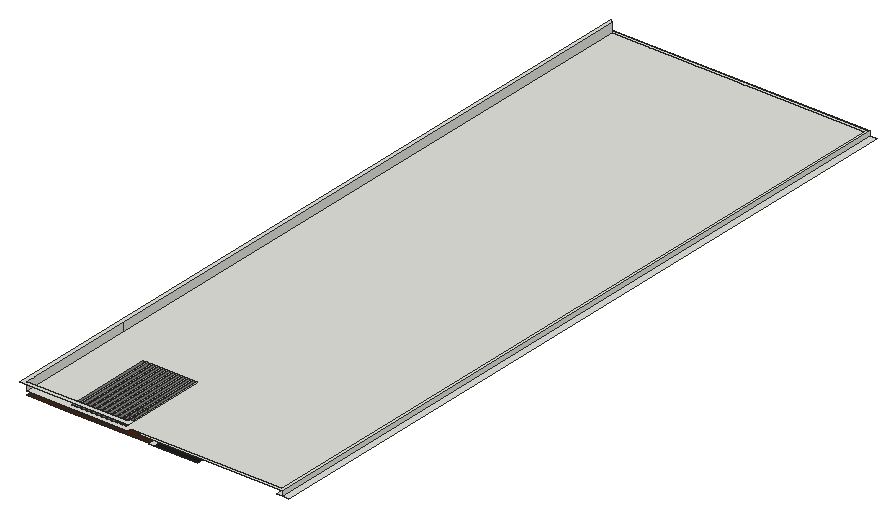
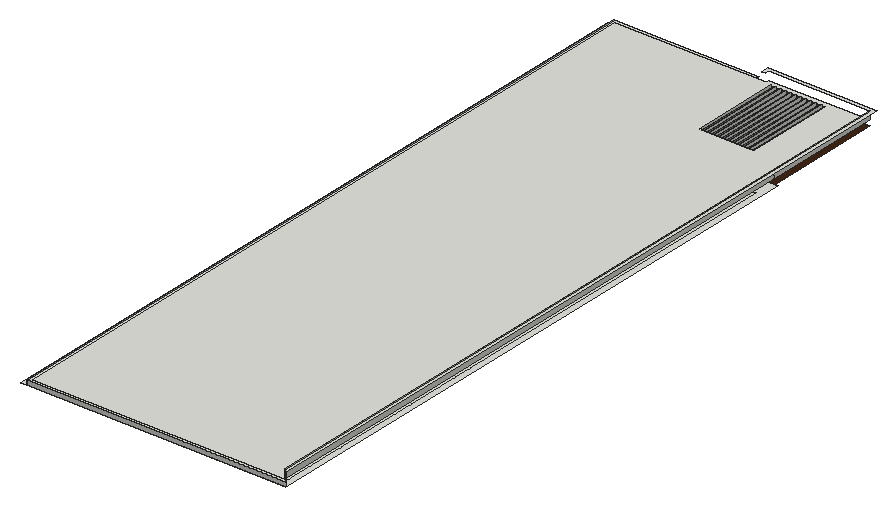
# SketchUp Ruby script. Lengths in inches.
U = 1.inch
M = Sketchup.active_model
def pt(a) = Geom::Point3d.new(a.map { |v| v * U })
def face(e, loops, mat)
  f = e.add_face(loops[0].map { |a| pt(a) })
  loops[1..].each { |l| e.add_face(l.map { |a| pt(a) }).erase! }
  f.material = f.back_material = mat if mat
  f
end
# faces: each face lists its corners as indices into pts; further lists are holes
def faces(e, pts, list, mat = nil) = list.each { |f| face(e, (f[0].is_a?(Array) ? f : [f]).map { |l| l.map { |i| pts[i] } }, mat) }
# xy, xz, yz: faces in a plane at the given z, y or x. An outline is a flat list of corners, or four numbers for a rectangle; further outlines are holes
def ring(l) = l.size == 4 ? [[l[0], l[1]], [l[2], l[1]], [l[2], l[3]], [l[0], l[3]]] : l.each_slice(2).to_a
def flat(e, list, mat, &to3) = list.each { |f| face(e, (f[0].is_a?(Array) ? f : [f]).map { |l| ring(l).map { |u, v| to3.(u, v) } }, mat) }
def xy(e, z, list, mat = nil) = flat(e, list, mat) { |x, y| [x, y, z] }
def xz(e, y, list, mat = nil) = flat(e, list, mat) { |x, z| [x, y, z] }
def yz(e, x, list, mat = nil) = flat(e, list, mat) { |y, z| [x, y, z] }
def lines(e, pts, list) = list.each { |a, b| e.add_line(pt(pts[a]), pt(pts[b])) }
# prism: a flat outline (further loops are holes) pulled along v
def prism(e, loops, v, mat = nil)
  f = face(e, loops, mat); d = Geom::Vector3d.new(v.map { |x| x * U })
  f.pushpull(f.normal.samedirection?(d) ? d.length : -d.length)
end
def box(e, o, s, mat = nil) = prism(e, [[o, [o[0] + s[0], o[1], o[2]], [o[0] + s[0], o[1] + s[1], o[2]], [o[0], o[1] + s[1], o[2]]]], [0, 0, s[2]], mat)
def at(x, y, z, deg = 0) = Geom::Transformation.translation(pt([x, y, z])) * Geom::Transformation.rotation(ORIGIN, Z_AXIS, deg.degrees)
def axes(o, x, y, z) = Geom::Transformation.new([*x, 0, *y, 0, *z, 0, *pt(o).to_a, 1])
def part(name) = M.definitions.add(name)
# library, detail: a bought-in or finely detailed component or shape, given as its bounding box
def library(name, o, s) = part(name).tap { |d| box(d.entities, o, s) }
def detail(e, o, s) = box(e.add_group.entities, o, s)
def put(e, d, t, mat = nil) = e.add_instance(d, t).tap { |i| i.material = mat if mat }
def group(e, t, mat = nil) = e.add_group.tap { |g| g.transformation = t; g.material = mat if mat }.entities
root = M.entities
M.materials.add("[Color M08]").color = [30, 30, 30]
M.materials.add("[Field Square Tile]").color = [211, 167, 108]
M.materials.add("[Granite Light Gray]").color = [149, 148, 144]
M.materials.add("[Wood Veneer 01]").color = [66, 38, 20]
xy(root,380.5,[[1555.29,2346.71,1555.29,3661.44,1107.53,3661.44,1107.53,2597.8,1323.53,2597.8,1323.53,2562.82,1097.72,2562.82,1097.72,3671.25,1565.1,3671.25,1565.1,2346.71],[1323.53,2346.71,1332.45,2425.46],[1565.1,2346.71,1576.91,3671.25],[1323.53,2425.46,1323.53,2597.8,1107.53,2597.8,1107.53,3661.44,1555.29,3661.44,1555.29,2425.46,1508.52,2425.46,1508.52,2532.83,1413.21,2532.83,1413.21,2573.65,1332.45,2573.65,1332.45,2532.83,1323.83,2532.83,1323.83,2425.46],[1323.83,2425.46,1332.45,2532.83],
  [1413.21,2425.46,1508.52,2532.83],[1332.45,2532.83,1413.21,2573.65]])
xy(root,380.5,[[1332.45,2346.71,1413.21,2532.83]],"[Color M08]")
xy(root,380.5,[[[1102.55,2347.9,1174.48,2562.82],[1119.58,2501.63,1121.1,2502.01,1122.48,2502.76,1123.61,2503.84,1124.42,2505.18,1124.85,2506.6875,1124.89,2508.25,1124.51,2509.78,1123.76,2511.15,1122.67,2512.28,1121.33,2513.09,1119.83,2513.53,1118.26,2513.56,1116.74,2513.19,1115.37,2512.43,1114.24,2511.35,1113.43,2510.01,1112.99,2508.5,1112.96,2506.9375,1113.33,2505.41,1114.09,2504.04,1115.17,2502.91,1116.51,2502.1,1118.02,2501.66],[1119.58,2441.63,1121.1,2442.01,1122.48,2442.76,1123.61,2443.84,1124.42,2445.18,1124.85,2446.6875,1124.89,2448.25,1124.51,2449.78,1123.76,2451.15,1122.67,2452.28,1121.33,2453.09,1119.83,2453.53,1118.26,2453.56,1116.74,2453.19,1115.37,2452.43,1114.24,2451.35,1113.43,2450.01,1112.99,2448.5,1112.96,2446.9375,1113.33,2445.41,1114.09,2444.04,1115.17,2442.91,1116.51,2442.1,1118.02,2441.66],[1119.58,2389.88,1121.1,2390.26,1122.48,2391.01,1123.61,2392.09,1124.42,2393.43,1124.85,2394.9375,1124.89,2396.5,1124.51,2398.03,1123.76,2399.4,1122.67,2400.53,1121.33,2401.34,1119.83,2401.78,1118.26,2401.81,1116.74,2401.44,1115.37,2400.68,1114.24,2399.6,1113.43,2398.26,1112.99,2396.75,1112.96,2395.1875,1113.33,2393.66,1114.09,2392.29,1115.17,2391.16,1116.51,2390.35,1118.02,2389.91],[1119.58,2359.13,1121.1,2359.51,1122.48,2360.26,1123.61,2361.34,1124.42,2362.68,1124.85,2364.1875,1124.89,2365.75,1124.51,2367.28,1123.76,2368.65,1122.67,2369.78,1121.33,2370.59,1119.83,2371.03,1118.26,2371.06,1116.74,2370.69,1115.37,2369.93,1114.24,2368.85,1113.43,2367.51,1112.99,2366,1112.96,2364.4375,1113.33,2362.91,1114.09,2361.54,1115.17,2360.41,1116.51,2359.6,1118.02,2359.16],[1159.33,2441.63,1160.85,2442.01,1162.23,2442.76,1163.36,2443.84,1164.17,2445.18,1164.6,2446.6875,1164.64,2448.25,1164.26,2449.78,1163.51,2451.15,1162.42,2452.28,1161.08,2453.09,1159.58,2453.53,1158.01,2453.56,1156.49,2453.19,1155.12,2452.43,1153.99,2451.35,1153.18,2450.01,1152.74,2448.5,1152.71,2446.9375,1153.08,2445.41,1153.84,2444.04,1154.92,2442.91,1156.26,2442.1,1157.77,2441.66],[1159.33,2389.88,1160.85,2390.26,1162.23,2391.01,1163.36,2392.09,1164.17,2393.43,1164.6,2394.9375,1164.64,2396.5,1164.26,2398.03,1163.51,2399.4,1162.42,2400.53,1161.08,2401.34,1159.58,2401.78,1158.01,2401.81,1156.49,2401.44,1155.12,2400.68,1153.99,2399.6,1153.18,2398.26,1152.74,2396.75,1152.71,2395.1875,1153.08,2393.66,1153.84,2392.29,1154.92,2391.16,1156.26,2390.35,1157.77,2389.91],[1159.33,2359.13,1160.85,2359.51,1162.23,2360.26,1163.36,2361.34,1164.17,2362.68,1164.6,2364.1875,1164.64,2365.75,1164.26,2367.28,1163.51,2368.65,1162.42,2369.78,1161.08,2370.59,1159.58,2371.03,1158.01,2371.06,1156.49,2370.69,1155.12,2369.93,1153.99,2368.85,1153.18,2367.51,1152.74,2366,1152.71,2364.4375,1153.08,2362.91,1153.84,2361.54,1154.92,2360.41,1156.26,2359.6,1157.77,2359.16],[1159.33,2501.63,1160.85,2502.01,1162.23,2502.76,1163.36,2503.84,1164.17,2505.18,1164.6,2506.6875,1164.64,2508.25,1164.26,2509.78,1163.51,2511.15,1162.42,2512.28,1161.08,2513.09,1159.58,2513.53,1158.01,2513.56,1156.49,2513.19,1155.12,2512.43,1153.99,2511.35,1153.18,2510.01,1152.74,2508.5,1152.71,2506.9375,1153.08,2505.41,1153.84,2504.04,1154.92,2502.91,1156.26,2502.1,1157.77,2501.66]],[[1174.48,2347.9,1323.53,2562.82],[1269.93,2355.06,1276.18,2516.12],[1260.81,2355.06,1267.06,2516.12],[1251.68,2355.06,1257.93,2516.12],[1242.56,2355.06,1248.81,2516.12],[1233.43,2355.06,1239.68,2516.12],[1224.31,2355.06,1230.56,2516.12],[1215.18,2355.06,1221.43,2516.12],[1206.06,2355.06,1212.31,2516.12],[1196.93,2355.06,1203.18,2516.12],[1187.81,2355.06,1194.06,2516.12],[1178.68,2355.06,1184.93,2516.12]]],"[Wood Veneer 01]")
xy(root,381.875,[[1119.58,2389.88,1118.02,2389.91,1116.51,2390.35,1115.17,2391.16,1114.09,2392.29,1113.33,2393.66,1112.96,2395.1875,1112.99,2396.75,1113.43,2398.26,1114.24,2399.6,1115.37,2400.68,1116.74,2401.44,1118.26,2401.81,1119.83,2401.78,1121.33,2401.34,1122.67,2400.53,1123.76,2399.4,1124.51,2398.03,1124.89,2396.5,1124.85,2394.9375,1124.42,2393.43,1123.61,2392.09,1122.48,2391.01,1121.1,2390.26],[1159.33,2389.88,1157.77,2389.91,1156.26,2390.35,1154.92,2391.16,1153.84,2392.29,1153.08,2393.66,1152.71,2395.1875,1152.74,2396.75,1153.18,2398.26,1153.99,2399.6,1155.12,2400.68,1156.49,2401.44,1158.01,2401.81,1159.58,2401.78,1161.08,2401.34,1162.42,2400.53,1163.51,2399.4,1164.26,2398.03,1164.64,2396.5,1164.6,2394.9375,1164.17,2393.43,1163.36,2392.09,1162.23,2391.01,1160.85,2390.26],[1119.58,2441.63,1118.02,2441.66,1116.51,2442.1,1115.17,2442.91,1114.09,2444.04,1113.33,2445.41,1112.96,2446.9375,1112.99,2448.5,1113.43,2450.01,1114.24,2451.35,1115.37,2452.43,1116.74,2453.19,1118.26,2453.56,1119.83,2453.53,1121.33,2453.09,1122.67,2452.28,1123.76,2451.15,1124.51,2449.78,1124.89,2448.25,1124.85,2446.6875,1124.42,2445.18,1123.61,2443.84,1122.48,2442.76,1121.1,2442.01],[1159.33,2441.63,1157.77,2441.66,1156.26,2442.1,1154.92,2442.91,1153.84,2444.04,1153.08,2445.41,1152.71,2446.9375,1152.74,2448.5,1153.18,2450.01,1153.99,2451.35,1155.12,2452.43,1156.49,2453.19,1158.01,2453.56,1159.58,2453.53,1161.08,2453.09,1162.42,2452.28,1163.51,2451.15,1164.26,2449.78,1164.64,2448.25,1164.6,2446.6875,1164.17,2445.18,1163.36,2443.84,1162.23,2442.76,1160.85,2442.01],[1119.58,2501.63,1118.02,2501.66,1116.51,2502.1,1115.17,2502.91,1114.09,2504.04,1113.33,2505.41,1112.96,2506.9375,1112.99,2508.5,1113.43,2510.01,1114.24,2511.35,1115.37,2512.43,1116.74,2513.19,1118.26,2513.56,1119.83,2513.53,1121.33,2513.09,1122.67,2512.28,1123.76,2511.15,1124.51,2509.78,1124.89,2508.25,1124.85,2506.6875,1124.42,2505.18,1123.61,2503.84,1122.48,2502.76,1121.1,2502.01],
  [1159.33,2501.63,1157.77,2501.66,1156.26,2502.1,1154.92,2502.91,1153.84,2504.04,1153.08,2505.41,1152.71,2506.9375,1152.74,2508.5,1153.18,2510.01,1153.99,2511.35,1155.12,2512.43,1156.49,2513.19,1158.01,2513.56,1159.58,2513.53,1161.08,2513.09,1162.42,2512.28,1163.51,2511.15,1164.26,2509.78,1164.64,2508.25,1164.6,2506.6875,1164.17,2505.18,1163.36,2503.84,1162.23,2502.76,1160.85,2502.01]],"[Field Square Tile]")
xy(root,388.625,[[[1104.06,2346.49,1287.38,2346.49,1287.38,2353.05,1558.75,2353.05,1558.75,3664.91,1104.06,3664.91],[1178.68,2355.06,1184.93,2516.12],[1187.81,2355.06,1194.06,2516.12],[1196.93,2355.06,1203.18,2516.12],[1206.06,2355.06,1212.31,2516.12],[1215.18,2355.06,1221.43,2516.12],[1224.31,2355.06,1230.56,2516.12],[1233.43,2355.06,1239.68,2516.12],[1242.56,2355.06,1248.81,2516.12],[1251.68,2355.06,1257.93,2516.12],[1260.81,2355.06,1267.06,2516.12],[1269.93,2355.06,1276.18,2516.12]],[1304.4375,2346.71,1565.1,2346.71,1565.1,3671.25,1097.72,3671.25,1104.06,3664.91,1558.75,3664.91,1558.75,2353.05,1304.4375,2353.05]])
xy(root,403.8125,[[1097.72,2340.15,1293.73,2340.15,1293.73,2353.05,1287.38,2353.05,1287.38,2346.49,1104.06,2346.49,1104.06,3664.91,1097.72,3671.25]])
xz(root,2516.12,[[1178.68,380.5,1184.93,388.625],[1187.81,380.5,1194.06,388.625],[1196.93,380.5,1203.18,388.625],[1206.06,380.5,1212.31,388.625],[1215.18,380.5,1221.43,388.625],
  [1224.31,380.5,1230.56,388.625],[1233.43,380.5,1239.68,388.625],[1242.56,380.5,1248.81,388.625],[1251.68,380.5,1257.93,388.625],[1260.81,380.5,1267.06,388.625],
  [1269.93,380.5,1276.18,388.625]],"[Granite Light Gray]")
xz(root,3671.25,[[1097.72,380.5,1565.1,388.625]])
yz(root,1104.06,[[2346.49,388.625,2562.82,403.8125],[2562.82,388.625,3664.91,403.8125]])
yz(root,1178.68,[[2355.06,380.5,2516.12,388.625]],"[Granite Light Gray]")
yz(root,1184.93,[[2355.06,380.5,2516.12,388.625]])
yz(root,1187.81,[[2355.06,380.5,2516.12,388.625]],"[Granite Light Gray]")
yz(root,1194.06,[[2355.06,380.5,2516.12,388.625]])
yz(root,1196.93,[[2355.06,380.5,2516.12,388.625]],"[Granite Light Gray]")
yz(root,1203.18,[[2355.06,380.5,2516.12,388.625]])
yz(root,1206.06,[[2355.06,380.5,2516.12,388.625]],"[Granite Light Gray]")
yz(root,1212.31,[[2355.06,380.5,2516.12,388.625]])
yz(root,1215.18,[[2355.06,380.5,2516.12,388.625]],"[Granite Light Gray]")
yz(root,1221.43,[[2355.06,380.5,2516.12,388.625]])
yz(root,1224.31,[[2355.06,380.5,2516.12,388.625]],"[Granite Light Gray]")
yz(root,1230.56,[[2355.06,380.5,2516.12,388.625]])
yz(root,1233.43,[[2355.06,380.5,2516.12,388.625]],"[Granite Light Gray]")
yz(root,1239.68,[[2355.06,380.5,2516.12,388.625]])
yz(root,1242.56,[[2355.06,380.5,2516.12,388.625]],"[Granite Light Gray]")
yz(root,1248.81,[[2355.06,380.5,2516.12,388.625]])
yz(root,1251.68,[[2355.06,380.5,2516.12,388.625]],"[Granite Light Gray]")
yz(root,1257.93,[[2355.06,380.5,2516.12,388.625]])
yz(root,1260.81,[[2355.06,380.5,2516.12,388.625]],"[Granite Light Gray]")
yz(root,1267.06,[[2355.06,380.5,2516.12,388.625]])
yz(root,1269.93,[[2355.06,380.5,2516.12,388.625]],"[Granite Light Gray]")
yz(root,1276.18,[[2355.06,380.5,2516.12,388.625]])
yz(root,1565.1,[[2346.71,380.5,3671.25,388.625]])
p = [[1118.26,2371.06,380.5],[1119.83,2371.03,380.5],[1119.83,2371.03,381.875],[1118.26,2371.06,381.875],[1158.01,2371.06,380.5],[1159.58,2371.03,380.5],
  [1159.58,2371.03,381.875],[1158.01,2371.06,381.875],[1118.02,2389.91,380.5],[1116.51,2390.35,380.5],[1116.51,2390.35,381.875],[1118.02,2389.91,381.875],
  [1119.58,2389.88,380.5],[1119.58,2389.88,381.875],[1121.1,2390.26,380.5],[1121.1,2390.26,381.875],[1157.77,2389.91,380.5],[1156.26,2390.35,380.5],
  [1156.26,2390.35,381.875],[1157.77,2389.91,381.875],[1159.33,2389.88,380.5],[1159.33,2389.88,381.875],[1160.85,2390.26,380.5],[1160.85,2390.26,381.875],
  [1122.48,2391.01,380.5],[1122.48,2391.01,381.875],[1162.23,2391.01,380.5],[1162.23,2391.01,381.875],[1115.17,2391.16,380.5],[1115.17,2391.16,381.875],
  [1154.92,2391.16,380.5],[1154.92,2391.16,381.875],[1123.61,2392.09,380.5],[1123.61,2392.09,381.875],[1163.36,2392.09,380.5],[1163.36,2392.09,381.875],
  [1114.09,2392.29,380.5],[1114.09,2392.29,381.875],[1153.84,2392.29,380.5],[1153.84,2392.29,381.875],[1124.42,2393.43,380.5],[1124.42,2393.43,381.875],
  [1164.17,2393.43,380.5],[1164.17,2393.43,381.875],[1113.33,2393.66,380.5],[1113.33,2393.66,381.875],[1153.08,2393.66,380.5],[1153.08,2393.66,381.875],
  [1124.85,2394.9375,380.5],[1124.85,2394.9375,381.875],[1164.6,2394.9375,380.5],[1164.6,2394.9375,381.875],[1112.96,2395.1875,380.5],[1112.96,2395.1875,381.875],
  [1152.71,2395.1875,380.5],[1152.71,2395.1875,381.875],[1124.89,2396.5,380.5],[1124.89,2396.5,381.875],[1164.64,2396.5,380.5],[1164.64,2396.5,381.875],
  [1112.99,2396.75,380.5],[1112.99,2396.75,381.875],[1152.74,2396.75,380.5],[1152.74,2396.75,381.875],[1124.51,2398.03,380.5],[1124.51,2398.03,381.875],
  [1164.26,2398.03,380.5],[1164.26,2398.03,381.875],[1113.43,2398.26,380.5],[1113.43,2398.26,381.875],[1153.18,2398.26,380.5],[1153.18,2398.26,381.875],
  [1123.76,2399.4,380.5],[1123.76,2399.4,381.875],[1163.51,2399.4,380.5],[1163.51,2399.4,381.875],[1114.24,2399.6,380.5],[1114.24,2399.6,381.875],
  [1153.99,2399.6,380.5],[1153.99,2399.6,381.875],[1122.67,2400.53,380.5],[1122.67,2400.53,381.875],[1162.42,2400.53,380.5],[1162.42,2400.53,381.875],
  [1115.37,2400.68,380.5],[1115.37,2400.68,381.875],[1155.12,2400.68,380.5],[1155.12,2400.68,381.875],[1121.33,2401.34,380.5],[1121.33,2401.34,381.875],
  [1161.08,2401.34,380.5],[1161.08,2401.34,381.875],[1116.74,2401.44,380.5],[1116.74,2401.44,381.875],[1156.49,2401.44,380.5],[1156.49,2401.44,381.875],
  [1119.83,2401.78,380.5],[1119.83,2401.78,381.875],[1159.58,2401.78,380.5],[1159.58,2401.78,381.875],[1118.26,2401.81,380.5],[1118.26,2401.81,381.875],
  [1158.01,2401.81,380.5],[1158.01,2401.81,381.875],[1119.58,2441.63,380.5],[1118.02,2441.66,380.5],[1118.02,2441.66,381.875],[1119.58,2441.63,381.875],
  [1121.1,2442.01,380.5],[1121.1,2442.01,381.875],[1159.33,2441.63,380.5],[1157.77,2441.66,380.5],[1157.77,2441.66,381.875],[1159.33,2441.63,381.875],
  [1160.85,2442.01,380.5],[1160.85,2442.01,381.875],[1116.51,2442.1,380.5],[1116.51,2442.1,381.875],[1156.26,2442.1,380.5],[1156.26,2442.1,381.875],
  [1122.48,2442.76,380.5],[1122.48,2442.76,381.875],[1162.23,2442.76,380.5],[1162.23,2442.76,381.875],[1115.17,2442.91,380.5],[1115.17,2442.91,381.875],
  [1154.92,2442.91,380.5],[1154.92,2442.91,381.875],[1123.61,2443.84,380.5],[1123.61,2443.84,381.875],[1163.36,2443.84,380.5],[1163.36,2443.84,381.875],
  [1114.09,2444.04,380.5],[1114.09,2444.04,381.875],[1153.84,2444.04,380.5],[1153.84,2444.04,381.875],[1124.42,2445.18,380.5],[1124.42,2445.18,381.875],
  [1164.17,2445.18,380.5],[1164.17,2445.18,381.875],[1113.33,2445.41,380.5],[1113.33,2445.41,381.875],[1153.08,2445.41,380.5],[1153.08,2445.41,381.875],
  [1124.85,2446.6875,380.5],[1124.85,2446.6875,381.875],[1164.6,2446.6875,380.5],[1164.6,2446.6875,381.875],[1112.96,2446.9375,380.5],[1112.96,2446.9375,381.875],
  [1152.71,2446.9375,380.5],[1152.71,2446.9375,381.875],[1124.89,2448.25,380.5],[1124.89,2448.25,381.875],[1164.64,2448.25,380.5],[1164.64,2448.25,381.875],
  [1112.99,2448.5,380.5],[1112.99,2448.5,381.875],[1152.74,2448.5,380.5],[1152.74,2448.5,381.875],[1124.51,2449.78,380.5],[1124.51,2449.78,381.875],
  [1164.26,2449.78,380.5],[1164.26,2449.78,381.875],[1113.43,2450.01,380.5],[1113.43,2450.01,381.875],[1153.18,2450.01,380.5],[1153.18,2450.01,381.875],
  [1123.76,2451.15,380.5],[1123.76,2451.15,381.875],[1163.51,2451.15,380.5],[1163.51,2451.15,381.875],[1114.24,2451.35,380.5],[1114.24,2451.35,381.875],
  [1153.99,2451.35,380.5],[1153.99,2451.35,381.875],[1122.67,2452.28,380.5],[1122.67,2452.28,381.875],[1162.42,2452.28,380.5],[1162.42,2452.28,381.875],
  [1115.37,2452.43,380.5],[1115.37,2452.43,381.875],[1155.12,2452.43,380.5],[1155.12,2452.43,381.875],[1121.33,2453.09,380.5],[1121.33,2453.09,381.875],
  [1161.08,2453.09,380.5],[1161.08,2453.09,381.875],[1116.74,2453.19,380.5],[1116.74,2453.19,381.875],[1156.49,2453.19,380.5],[1156.49,2453.19,381.875],
  [1119.83,2453.53,380.5],[1119.83,2453.53,381.875],[1159.58,2453.53,380.5],[1159.58,2453.53,381.875],[1118.26,2453.56,380.5],[1118.26,2453.56,381.875],
  [1158.01,2453.56,380.5],[1158.01,2453.56,381.875],[1119.58,2501.63,380.5],[1118.02,2501.66,380.5],[1118.02,2501.66,381.875],[1119.58,2501.63,381.875],
  [1121.1,2502.01,380.5],[1121.1,2502.01,381.875],[1159.33,2501.63,380.5],[1157.77,2501.66,380.5],[1157.77,2501.66,381.875],[1159.33,2501.63,381.875],
  [1160.85,2502.01,380.5],[1160.85,2502.01,381.875],[1116.51,2502.1,380.5],[1116.51,2502.1,381.875],[1156.26,2502.1,380.5],[1156.26,2502.1,381.875],
  [1122.48,2502.76,380.5],[1122.48,2502.76,381.875],[1162.23,2502.76,380.5],[1162.23,2502.76,381.875],[1115.17,2502.91,380.5],[1115.17,2502.91,381.875],
  [1154.92,2502.91,380.5],[1154.92,2502.91,381.875],[1123.61,2503.84,380.5],[1123.61,2503.84,381.875],[1163.36,2503.84,380.5],[1163.36,2503.84,381.875],
  [1114.09,2504.04,380.5],[1114.09,2504.04,381.875],[1153.84,2504.04,380.5],[1153.84,2504.04,381.875],[1124.42,2505.18,380.5],[1124.42,2505.18,381.875],
  [1164.17,2505.18,380.5],[1164.17,2505.18,381.875],[1113.33,2505.41,380.5],[1113.33,2505.41,381.875],[1153.08,2505.41,380.5],[1153.08,2505.41,381.875],
  [1124.85,2506.6875,380.5],[1124.85,2506.6875,381.875],[1164.6,2506.6875,380.5],[1164.6,2506.6875,381.875],[1112.96,2506.9375,380.5],[1112.96,2506.9375,381.875],
  [1152.71,2506.9375,380.5],[1152.71,2506.9375,381.875],[1124.89,2508.25,380.5],[1124.89,2508.25,381.875],[1164.64,2508.25,380.5],[1164.64,2508.25,381.875],
  [1112.99,2508.5,380.5],[1112.99,2508.5,381.875],[1152.74,2508.5,380.5],[1152.74,2508.5,381.875],[1124.51,2509.78,380.5],[1124.51,2509.78,381.875],
  [1164.26,2509.78,380.5],[1164.26,2509.78,381.875],[1113.43,2510.01,380.5],[1113.43,2510.01,381.875],[1153.18,2510.01,380.5],[1153.18,2510.01,381.875],
  [1123.76,2511.15,380.5],[1123.76,2511.15,381.875],[1163.51,2511.15,380.5],[1163.51,2511.15,381.875],[1114.24,2511.35,380.5],[1114.24,2511.35,381.875],
  [1153.99,2511.35,380.5],[1153.99,2511.35,381.875],[1122.67,2512.28,380.5],[1122.67,2512.28,381.875],[1162.42,2512.28,380.5],[1162.42,2512.28,381.875],
  [1115.37,2512.43,380.5],[1115.37,2512.43,381.875],[1155.12,2512.43,380.5],[1155.12,2512.43,381.875],[1121.33,2513.09,380.5],[1121.33,2513.09,381.875],
  [1161.08,2513.09,380.5],[1161.08,2513.09,381.875],[1116.74,2513.19,380.5],[1116.74,2513.19,381.875],[1156.49,2513.19,380.5],[1156.49,2513.19,381.875],
  [1119.83,2513.53,380.5],[1119.83,2513.53,381.875],[1159.58,2513.53,380.5],[1159.58,2513.53,381.875],[1118.26,2513.56,380.5],[1118.26,2513.56,381.875],
  [1158.01,2513.56,380.5],[1158.01,2513.56,381.875],[1104.06,3664.91,388.625],[1097.72,3671.25,388.625],[1097.72,3671.25,403.8125],[1104.06,3664.91,403.8125]]
faces(root,p,[[0,1,2,3],[4,5,6,7],[8,9,10,11],[12,8,11,13],[14,12,13,15],[16,17,18,19],[20,16,19,21],[22,20,21,23],
  [24,14,15,25],[26,22,23,27],[9,28,29,10],[17,30,31,18],[32,24,25,33],[34,26,27,35],[28,36,37,29],[30,38,39,31],
  [40,32,33,41],[42,34,35,43],[36,44,45,37],[38,46,47,39],[48,40,41,49],[50,42,43,51],[44,52,53,45],[46,54,55,47],
  [56,48,49,57],[58,50,51,59],[52,60,61,53],[54,62,63,55],[64,56,57,65],[66,58,59,67],[60,68,69,61],[62,70,71,63],
  [72,64,65,73],[74,66,67,75],[68,76,77,69],[70,78,79,71],[80,72,73,81],[82,74,75,83],[76,84,85,77],[78,86,87,79],
  [88,80,81,89],[90,82,83,91],[84,92,93,85],[86,94,95,87],[96,88,89,97],[98,90,91,99],[92,100,101,93],[94,102,103,95],
  [100,96,97,101],[102,98,99,103],[104,105,106,107],[108,104,107,109],[110,111,112,113],[114,110,113,115],[105,116,117,106],[111,118,119,112],
  [120,108,109,121],[122,114,115,123],[116,124,125,117],[118,126,127,119],[128,120,121,129],[130,122,123,131],[124,132,133,125],[126,134,135,127],
  [136,128,129,137],[138,130,131,139],[132,140,141,133],[134,142,143,135],[144,136,137,145],[146,138,139,147],[140,148,149,141],[142,150,151,143],
  [152,144,145,153],[154,146,147,155],[148,156,157,149],[150,158,159,151],[160,152,153,161],[162,154,155,163],[156,164,165,157],[158,166,167,159],
  [168,160,161,169],[170,162,163,171],[164,172,173,165],[166,174,175,167],[176,168,169,177],[178,170,171,179],[172,180,181,173],[174,182,183,175],
  [184,176,177,185],[186,178,179,187],[180,188,189,181],[182,190,191,183],[192,184,185,193],[194,186,187,195],[188,196,197,189],[190,198,199,191],
  [196,192,193,197],[198,194,195,199],[200,201,202,203],[204,200,203,205],[206,207,208,209],[210,206,209,211],[201,212,213,202],[207,214,215,208],
  [216,204,205,217],[218,210,211,219],[212,220,221,213],[214,222,223,215],[224,216,217,225],[226,218,219,227],[220,228,229,221],[222,230,231,223],
  [232,224,225,233],[234,226,227,235],[228,236,237,229],[230,238,239,231],[240,232,233,241],[242,234,235,243],[236,244,245,237],[238,246,247,239],
  [248,240,241,249],[250,242,243,251],[244,252,253,245],[246,254,255,247],[256,248,249,257],[258,250,251,259],[252,260,261,253],[254,262,263,255],
  [264,256,257,265],[266,258,259,267],[260,268,269,261],[262,270,271,263],[272,264,265,273],[274,266,267,275],[268,276,277,269],[270,278,279,271],
  [280,272,273,281],[282,274,275,283],[276,284,285,277],[278,286,287,279],[288,280,281,289],[290,282,283,291],[284,292,293,285],[286,294,295,287],
  [292,288,289,293],[294,290,291,295]],"[Field Square Tile]")
faces(root,p,[[296,297,298,299]])
